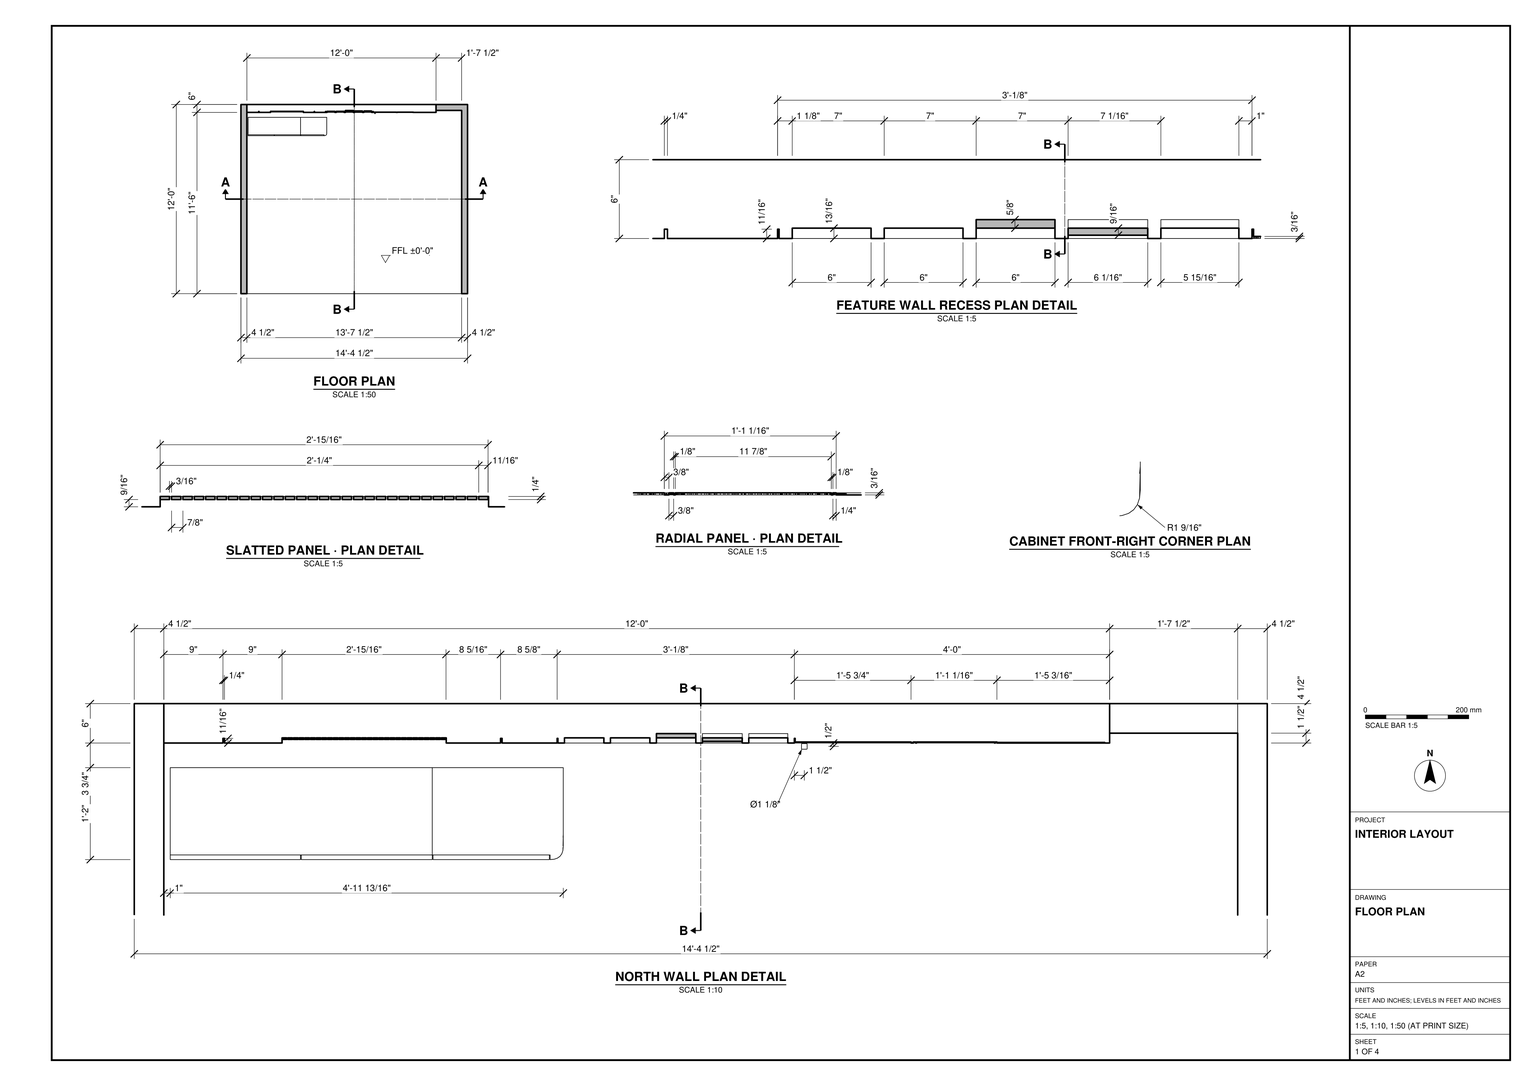
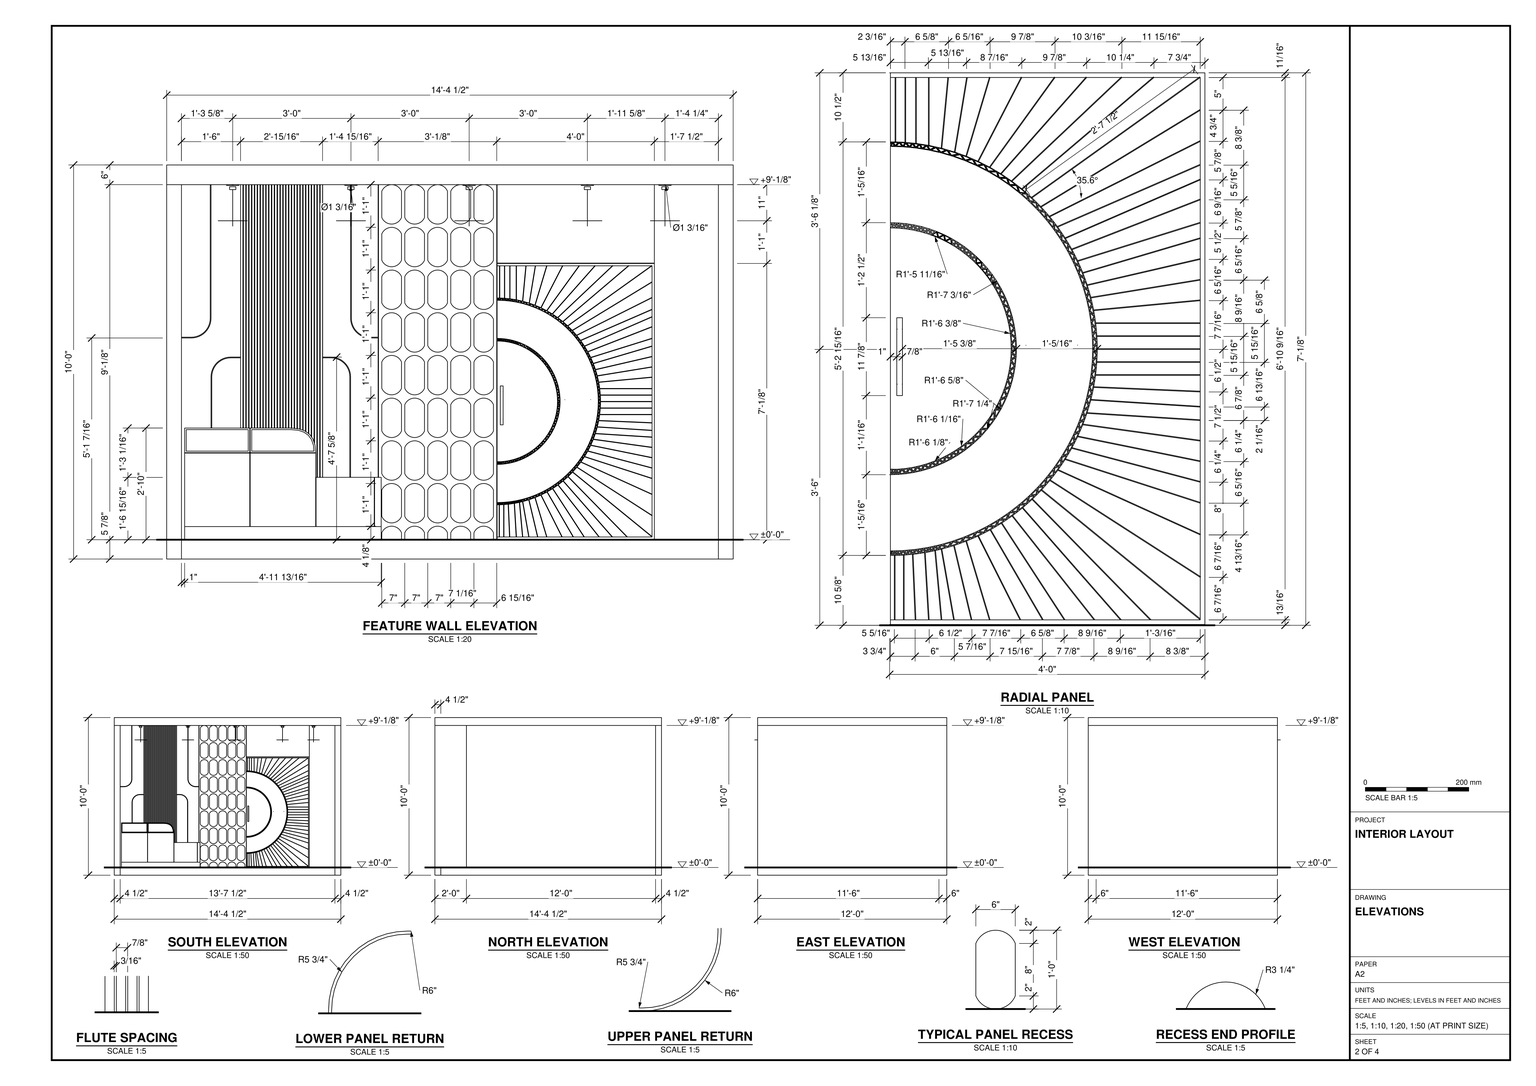
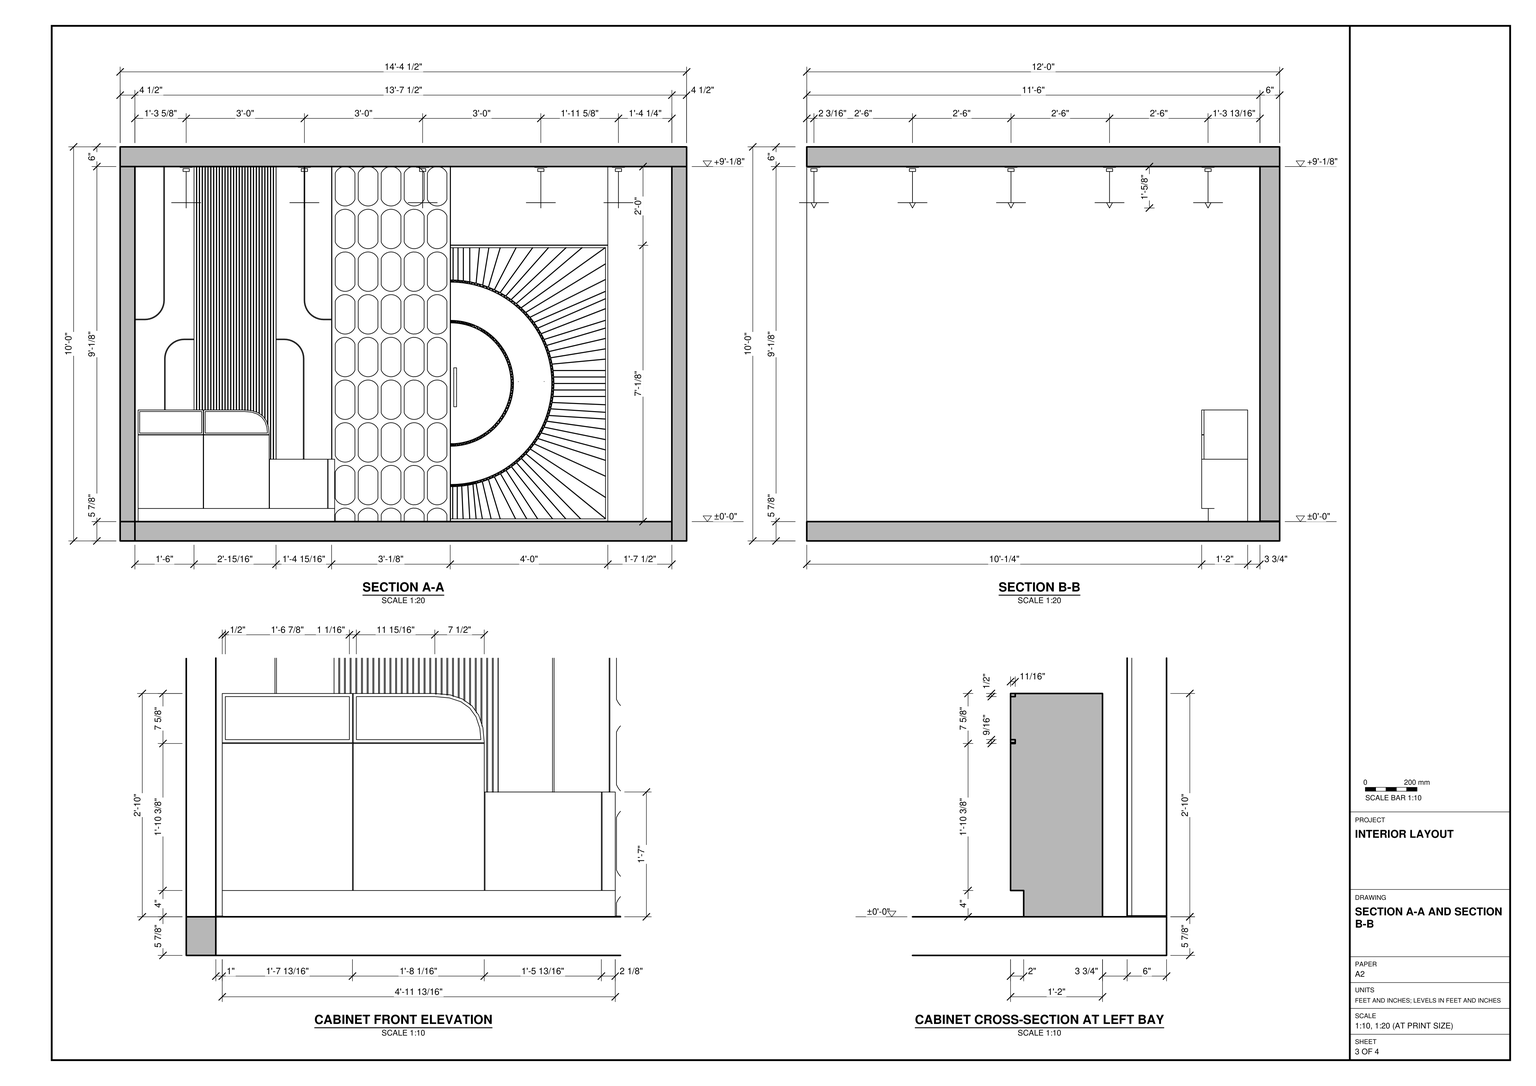
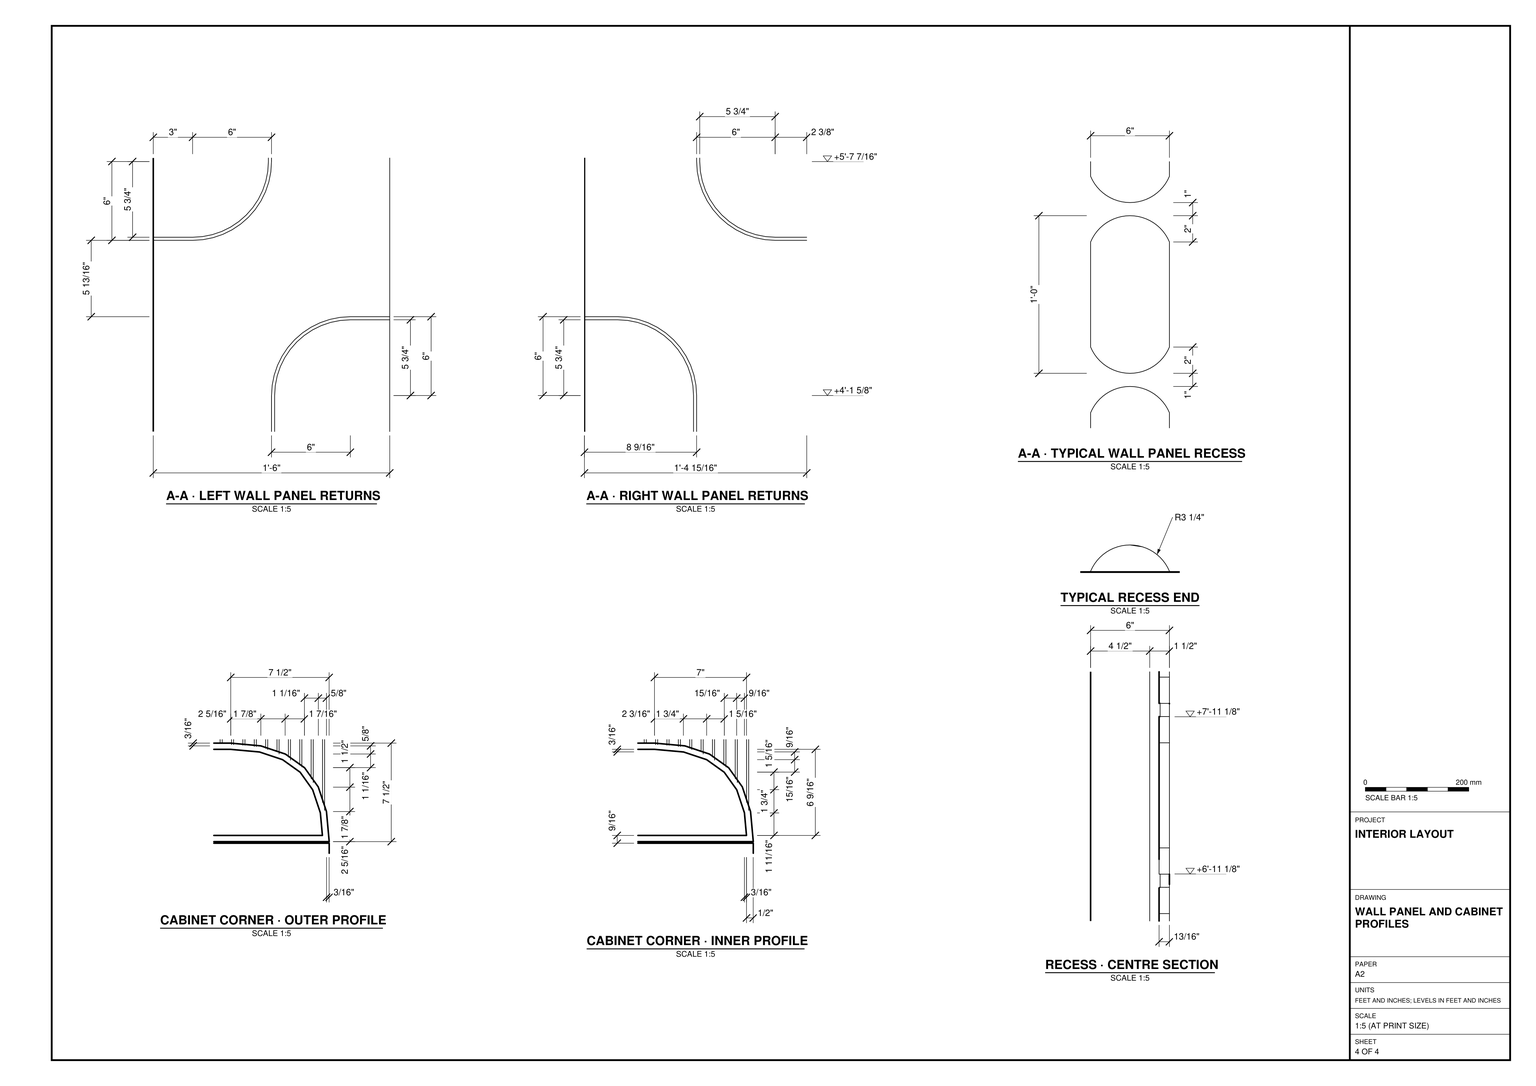
Build the interior in SketchUp from task_files/diagram_01.pdf. Work in feet and inches. The room shell is 14'-4 1/2" wide, 12'-0" deep and 10'-0" high overall, with the finished floor at ±0'-0". Model the floor slab, ceiling slab, north wall and two side walls at the thicknesses shown in plan and section. Leave the south side open so the feature wall can be seen in elevation.

Lay out the north wall from left to right. Model the narrow vertical slats and the curved returns of the adjacent panels, followed by the grid of rounded-ended recesses. Use the plan details to give these features depth. To the right of the recesses, fit the rectangular radial panel with its semicircular centre, surrounding band and divisions fanning out to the frame. Retain the plain wall above the radial panel and at its right end.

Place the stepped cabinet in front of the left-hand panels. Follow the cabinet details for its bay divisions, curved corner, recessed plinth and clearance from the wall. Position the lights as indicated in the sections. Lights, decor and loose items shown may use any suitable library components. Keep the shell elements and individual joinery pieces in separate groups or components, using components for repeated parts. Save one SketchUp model as output_files/room_with_a_feature_wall_and_stepped_cabinet.skp.

# SketchUp Ruby script. Lengths in inches.
U = 1.inch
M = Sketchup.active_model
def pt(a) = Geom::Point3d.new(a.map { |v| v * U })
def face(e, loops, mat)
  f = e.add_face(loops[0].map { |a| pt(a) })
  loops[1..].each { |l| e.add_face(l.map { |a| pt(a) }).erase! }
  f.material = f.back_material = mat if mat
  f
end
# faces: each face lists its corners as indices into pts; further lists are holes
def faces(e, pts, list, mat = nil) = list.each { |f| face(e, (f[0].is_a?(Array) ? f : [f]).map { |l| l.map { |i| pts[i] } }, mat) }
# xy, xz, yz: faces in a plane at the given z, y or x. An outline is a flat list of corners, or four numbers for a rectangle; further outlines are holes
def ring(l) = l.size == 4 ? [[l[0], l[1]], [l[2], l[1]], [l[2], l[3]], [l[0], l[3]]] : l.each_slice(2).to_a
def flat(e, list, mat, &to3) = list.each { |f| face(e, (f[0].is_a?(Array) ? f : [f]).map { |l| ring(l).map { |u, v| to3.(u, v) } }, mat) }
def xy(e, z, list, mat = nil) = flat(e, list, mat) { |x, y| [x, y, z] }
def xz(e, y, list, mat = nil) = flat(e, list, mat) { |x, z| [x, y, z] }
def yz(e, x, list, mat = nil) = flat(e, list, mat) { |y, z| [x, y, z] }
def lines(e, pts, list) = list.each { |a, b| e.add_line(pt(pts[a]), pt(pts[b])) }
# prism: a flat outline (further loops are holes) pulled along v
def prism(e, loops, v, mat = nil)
  f = face(e, loops, mat); d = Geom::Vector3d.new(v.map { |x| x * U })
  f.pushpull(f.normal.samedirection?(d) ? d.length : -d.length)
end
def box(e, o, s, mat = nil) = prism(e, [[o, [o[0] + s[0], o[1], o[2]], [o[0] + s[0], o[1] + s[1], o[2]], [o[0], o[1] + s[1], o[2]]]], [0, 0, s[2]], mat)
def at(x, y, z, deg = 0) = Geom::Transformation.translation(pt([x, y, z])) * Geom::Transformation.rotation(ORIGIN, Z_AXIS, deg.degrees)
def axes(o, x, y, z) = Geom::Transformation.new([*x, 0, *y, 0, *z, 0, *pt(o).to_a, 1])
def part(name) = M.definitions.add(name)
# library, detail: a bought-in or finely detailed component or shape, given as its bounding box
def library(name, o, s) = part(name).tap { |d| box(d.entities, o, s) }
def detail(e, o, s) = box(e.add_group.entities, o, s)
def put(e, d, t, mat = nil) = e.add_instance(d, t).tap { |i| i.material = mat if mat }
def group(e, t, mat = nil) = e.add_group.tap { |g| g.transformation = t; g.material = mat if mat }.entities
root = M.entities
M.materials.add("Tafisa-Gardenia-or-Gardenia-PM775-4K").color = [246, 245, 235]
M.materials.add("Uniboard-L19-Putty-4K").color = [187, 181, 160]
M.materials.add("[Color M09]").color = [0, 0, 0]
c1 = part("Group194\#1")
p = [[0,0,0],[0,0,-16.77],[-0.04,0,-16.77],[0.28,-54,0],[-0.28,-54,0],[0.28,54,0],
  [0.28,0,0],[-0.28,54,0],[0.04,0,-16.77],[-0.28,0,0],[0,0,-27.14]]
lines(c1.entities,p,[[0,1],[1,2],[3,4],[5,6],[7,5],[1,8],[9,0],[0,6],[8,10],[4,9],[6,3],[2,10],
  [9,7]])
c2 = part("Rectangle Light")
put(c2.entities,c1,at(0,0,0))
c3 = part("Group196\#1")
p = [[0,0,0],[0,0,-16.77],[-0.04,0,-16.77],[0.28,-54,0],[-0.28,-54,0],[0.28,54,0],
  [0.28,0,0],[-0.28,54,0],[0.04,0,-16.77],[-0.28,0,0],[0,0,-27.14]]
lines(c3.entities,p,[[0,1],[1,2],[3,4],[5,6],[7,5],[1,8],[9,0],[0,6],[8,10],[4,9],[6,3],[2,10],
  [9,7]])
c4 = part("Rectangle Light\#1")
put(c4.entities,c3,at(0,0,0))
c5 = library("Group",[0,0,0],[144,6,108])
c6 = library("Group\#8",[0,0,0],[8.9,8.9,12.62])
put(root,c2,axes([22.51,138.28,60],[0,-1,0],[0,0,-1],[-1,0,0]))
put(root,c4,axes([47.49,138.28,60],[0,-1,0],[0,0,-1],[1,0,0]))
g1 = group(root,at(4.5,0,0),"Tafisa-Gardenia-or-Gardenia-PM775-4K")
xy(g1,0,[[-4.5,0,0,144],[0,0,163.5,144],[163.5,0,168,144]])
xy(g1,5.88,[[-4.5,0,0,144],[0,0,163.5,0,163.5,139.5,144,139.5,144,144,0,144],[144,139.5,163.5,144]])
xy(g1,114,[[163.5,0,168,0,168,144,144,144,144,139.5,163.5,139.5]])
xz(g1,0,[[-4.5,0,0,5.88],[0,0,163.5,5.88],[163.5,0,168,114]])
xz(g1,139.5,[[144,5.88,163.5,114]])
xz(g1,144,[[-4.5,0,0,5.88],[0,0,163.5,5.88],[163.5,0,163.5,5.88,144,5.88,144,114,168,114,168,0]])
yz(g1,-4.5,[[0,0,144,5.88]])
yz(g1,0,[[0,0,144,5.88]])
yz(g1,144,[[139.5,5.88,144,114]])
yz(g1,163.5,[[0,0,144,5.88],[0,5.88,139.5,114]])
yz(g1,168,[[0,0,144,114]])
put(root,c5,at(4.5,138,6))
g2 = group(root,at(101.59,137.06,52.7))
xy(g2,-11.84,[[0.09,0,0.04,0.01,0.01,0.04,0,0.09,0,0.77,0.01,0.8125,0.04,0.85,0.09,0.86,0.77,0.86,0.8125,0.85,0.85,0.8125,0.86,0.77,0.86,0.09,0.85,0.04,0.81,0.01,0.77,0]],"[Color M09]")
xy(g2,-10.1,[[0,0.45,0.86,0.45,0.86,0.77,0.85,0.8125,0.8125,0.85,0.77,0.86,0.09,0.86,0.04,0.85,0.01,0.8125,0,0.77]],"[Color M09]")
xy(g2,-1.72,[[0,0.45,0,0.77,0.01,0.8125,0.04,0.85,0.09,0.86,0.77,0.86,0.8125,0.85,0.85,0.8125,0.86,0.77,0.86,0.45]],"[Color M09]")
xy(g2,0.02,[[0.09,0,0.77,0,0.81,0.01,0.85,0.04,0.86,0.09,0.86,0.77,0.85,0.8125,0.8125,0.85,0.77,0.86,0.09,0.86,0.04,0.85,0.01,0.8125,0,0.77,0,0.09,0.01,0.04,0.04,0.01]],"[Color M09]")
xz(g2,0,[[0.09,-11.84,0.77,0.02]],"[Color M09]")
xz(g2,0.26,[[0,-9.91,0.86,-1.91]],"[Color M09]")
xz(g2,0.86,[[0.09,-11.84,0.77,-10.1],[0.09,-1.72,0.77,0.02]],"[Color M09]")
yz(g2,0,[[0.09,-11.84,0.09,0.02,0.77,0.02,0.77,-1.72,0.45,-1.72,0.36,-1.75,0.29,-1.82,0.26,-1.91,0.26,-9.91,0.29,-10.01,0.36,-10.07,0.45,-10.1,0.77,-10.1,0.77,-11.84]],"[Color M09]")
yz(g2,0.86,[[0.09,-11.84,0.77,-11.84,0.77,-10.1,0.45,-10.1,0.36,-10.07,0.29,-10.01,0.26,-9.91,0.26,-1.91,0.29,-1.82,0.36,-1.75,0.45,-1.72,0.77,-1.72,0.77,0.02,0.09,0.02]],"[Color M09]")
p = [[0.04,0.01,-11.84],[0.09,0,-11.84],[0.09,0,0.02],[0.04,0.01,0.02],[0.01,0.04,-11.84],[0.01,0.04,0.02],
  [0,0.09,0.02],[0,0.09,-11.84],[0.85,0.04,-11.84],[0.85,0.04,0.02],[0.81,0.01,0.02],[0.81,0.01,-11.84],
  [0.77,0,-11.84],[0.77,0,0.02],[0.86,0.09,-11.84],[0.86,0.09,0.02],[0.01,0.8125,-11.84],[0,0.77,-11.84],
  [0,0.77,-10.1],[0.01,0.8125,-10.1],[0.04,0.85,-11.84],[0.04,0.85,-10.1],[0.09,0.86,-11.84],[0.09,0.86,-10.1],
  [0.8125,0.85,-11.84],[0.77,0.86,-11.84],[0.77,0.86,-10.1],[0.8125,0.85,-10.1],[0.85,0.8125,-11.84],[0.85,0.8125,-10.1],
  [0.86,0.77,-11.84],[0.86,0.77,-10.1],[0.86,0.29,-10.01],[0.86,0.36,-10.07],[0,0.36,-10.07],[0,0.29,-10.01],
  [0.86,0.45,-10.1],[0,0.45,-10.1],[0.86,0.26,-9.91],[0,0.26,-9.91],[0,0.29,-1.82],[0.86,0.29,-1.82],
  [0.86,0.26,-1.91],[0,0.26,-1.91],[0.86,0.36,-1.75],[0,0.36,-1.75],[0.86,0.45,-1.72],[0,0.45,-1.72],
  [0,0.77,-1.72],[0,0.77,0.02],[0.01,0.8125,0.02],[0.01,0.8125,-1.72],[0.04,0.85,0.02],[0.09,0.86,0.02],
  [0.09,0.86,-1.72],[0.04,0.85,-1.72],[0.77,0.86,0.02],[0.8125,0.85,0.02],[0.8125,0.85,-1.72],[0.77,0.86,-1.72],
  [0.85,0.8125,-1.72],[0.85,0.8125,0.02],[0.86,0.77,0.02],[0.86,0.77,-1.72]]
faces(g2,p,[[0,1,2,3],[4,0,3,5],[4,5,6,7],[8,9,10,11],[12,11,10,13],[14,15,9,8],[16,17,18,19],[20,16,19,21],
  [22,20,21,23],[24,25,26,27],[28,24,27,29],[30,28,29,31],[32,33,34,35],[33,36,37,34],[38,32,35,39],[40,41,42,43],
  [44,41,40,45],[46,44,45,47],[48,49,50,51],[52,53,54,55],[51,50,52,55],[56,57,58,59],[60,61,62,63],[57,61,60,58]],"[Color M09]")
g3 = group(root,at(0,0,5.88))
box(g3,[0,0,0],[4.5,144,108.12])
g4 = group(root,at(5.48,120.25,5.88),"Tafisa-Gardenia-or-Gardenia-PM775-4K")
xy(g4,0,[[0,2,0,14,59.84,14,59.84,3.8125,59.79,3.26,59.64,2.81,59.39,2.45,59.03,2.2,58.58,2.05,58.02,2]])
xy(g4,4,[[0,0,0,2,19.95,2,19.95,0.71,19.83,0.71,19.83,0],[19.95,0,39.89,0.71],[57.84,0,57.84,0.71,39.89,0.71,39.89,2,58.02,2,58.58,2.05,59.03,2.2,59.39,2.45,59.64,2.81,59.79,3.26,59.84,3.8125,59.78,1.39,59.62,0.89,59.34,0.5,58.95,0.22,58.45,0.06],[40.01,0,57.72,0.71],[19.95,0.71,39.89,2]])
xy(g4,19,[[40.01,0,57.72,0.71]])
xy(g4,19,[[57.84,0,58.45,0.06,58.95,0.22,59.34,0.5,59.62,0.89,59.78,1.39,59.84,2,59.84,14,39.89,14,39.89,0.71,57.84,0.71]],"Uniboard-L19-Putty-4K")
xy(g4,26.38,[[0,0,19.83,0.71],[19.95,0,39.89,0.71]])
xy(g4,26.5,[[0,0,19.83,0.71],[19.95,0,39.89,0.71]])
xy(g4,26.97,[[0.47,0,19.36,0.71],[20.42,0,39.375,0.71]])
xy(g4,33.53,[[0.47,0,19.36,0.71],[20.42,0,32.37,0.71]])
xy(g4,34,[[0,0,19.83,0.71],[19.95,0,32.39,0.71]])
xy(g4,34,[[0,0.71,32.39,14]],"Uniboard-L19-Putty-4K")
xz(g4,0,[[0,4,19.83,26.38],[19.95,4,39.89,26.38],[40.01,4,57.72,19],[0.47,26.97,19.36,33.53],[20.42,26.97,39.375,26.97,39.22,28.69,38.63,30.45,37.68,31.79,36.34,32.74,34.59,33.33,32.37,33.53,20.42,33.53]])
xz(g4,0,[[[0,26.5,19.83,34],[0.47,26.97,19.36,33.53]],[[19.95,26.5,39.89,26.5,39.68,28.79,39.06,30.67,38.02,32.125,36.56,33.17,34.68,33.79,32.39,34,19.95,34],[20.42,26.97,20.42,33.53,32.37,33.53,34.59,33.33,36.34,32.74,37.68,31.79,38.63,30.45,39.22,28.69,39.375,26.97]]],"Uniboard-L19-Putty-4K")
xz(g4,0.71,[[19.83,4,19.95,26.38],[19.95,4,39.89,26.38],[39.89,4,40.01,19],[40.01,4,57.72,19],[57.72,4,57.84,19],
  [0,26.38,19.95,26.5],[19.95,26.38,39.89,26.5],[[0,26.5,19.83,34],[0.47,26.97,19.36,33.53]],[[19.95,26.5,19.95,34,32.39,34,34.68,33.79,36.56,33.17,38.02,32.125,39.06,30.67,39.68,28.79,39.89,26.5],[20.42,26.97,39.375,26.97,39.22,28.69,38.63,30.45,37.68,31.79,36.34,32.74,34.59,33.33,32.37,33.53,20.42,33.53]]])
xz(g4,0.71,[[19.83,26.5,19.95,34]],"Uniboard-L19-Putty-4K")
xz(g4,2,[[0,0,58.02,4]],"Uniboard-L19-Putty-4K")
xz(g4,14,[[0,0,0,34,32.39,34,34.68,33.79,36.56,33.17,38.02,32.125,39.06,30.67,39.68,28.79,39.89,26.5,39.89,19,59.84,19,59.84,0]])
yz(g4,0,[[2,0,2,4,0,4,0,26.38,0.71,26.38,0.71,34,14,34,14,0],[0,26.5,0.71,34]])
yz(g4,0.47,[[0,26.97,0.71,33.53]])
yz(g4,19.36,[[0,26.97,0.71,33.53]])
yz(g4,19.83,[[0,4,0.71,26.38]])
yz(g4,19.83,[[0,26.5,0.71,34]],"Uniboard-L19-Putty-4K")
yz(g4,19.95,[[0,4,0.71,26.38],[0,26.5,0.71,34]])
yz(g4,20.42,[[0,26.97,0.71,33.53]])
yz(g4,39.89,[[0,4,0.71,19],[0,19,0.71,26.38]])
yz(g4,39.89,[[0.71,19,14,26.5]],"Uniboard-L19-Putty-4K")
yz(g4,40.01,[[0,4,0.71,19]])
yz(g4,57.72,[[0,4,0.71,19]])
yz(g4,57.84,[[0,4,0.71,19]])
yz(g4,59.84,[[3.8125,0,14,0,14,19,2,19,2,4,3.8125,4]],"Uniboard-L19-Putty-4K")
p = [[58.58,2.05,0],[58.58,2.05,4],[58.02,2,4],[58.02,2,0],[59.03,2.2,0],[59.03,2.2,4],
  [59.39,2.45,0],[59.39,2.45,4],[59.64,2.81,0],[59.64,2.81,4],[59.79,3.26,0],[59.79,3.26,4],
  [59.84,3.8125,0],[59.84,3.8125,4],[57.84,0,19],[57.84,0,4],[58.45,0.06,4],[58.45,0.06,19],
  [58.95,0.22,4],[58.95,0.22,19],[59.34,0.5,4],[59.34,0.5,19],[59.62,0.89,4],[59.62,0.89,19],
  [59.78,1.39,4],[59.78,1.39,19],[59.84,2,4],[59.84,2,19],[39.68,0.71,28.79],[39.68,0,28.79],
  [39.89,0,26.5],[39.89,0.71,26.5],[39.68,14,28.79],[39.89,14,26.5],[39.375,0.71,26.97],[39.375,0,26.97],
  [39.22,0,28.69],[39.22,0.71,28.69],[38.63,0,30.45],[38.63,0.71,30.45],[39.06,0.71,30.67],[39.06,0,30.67],
  [39.06,14,30.67],[37.68,0,31.79],[37.68,0.71,31.79],[38.02,0.71,32.125],[38.02,0,32.125],[38.02,14,32.125],
  [36.34,0,32.74],[36.34,0.71,32.74],[36.56,0.71,33.17],[36.56,0,33.17],[36.56,14,33.17],[34.59,0,33.33],
  [34.59,0.71,33.33],[34.68,0.71,33.79],[34.68,0,33.79],[34.68,14,33.79],[32.37,0,33.53],[32.37,0.71,33.53],
  [32.39,0.71,34],[32.39,0,34],[32.39,14,34]]
faces(g4,p,[[0,1,2,3],[4,5,1,0],[6,7,5,4],[8,9,7,6],[10,11,9,8],[12,13,11,10],[14,15,16,17],[17,16,18,19],
  [19,18,20,21],[21,20,22,23],[23,22,24,25],[25,24,26,27],[32,28,31,33],[42,40,28,32],[47,45,40,42],[52,50,45,47],
  [57,55,50,52],[62,60,55,57]],"Uniboard-L19-Putty-4K")
faces(g4,p,[[28,29,30,31],[34,35,36,37],[37,36,38,39],[40,41,29,28],[39,38,43,44],[45,46,41,40],[44,43,48,49],[50,51,46,45],
  [49,48,53,54],[55,56,51,50],[54,53,58,59],[60,61,56,55]])
g5 = group(root,at(0,0,114))
box(g5,[0,0,0],[172.5,144,6])
put(root,c6,at(15.66,117.74,101.38))
put(root,c6,at(51.66,117.74,101.38))
put(root,c6,at(87.66,117.74,101.38))
put(root,c6,at(123.66,117.74,101.38))
put(root,c6,at(147.28,117.74,101.38))
put(root,c6,at(51.66,87.74,101.38))
put(root,c6,at(123.66,87.74,101.38))
put(root,c6,at(15.66,87.74,101.38))
put(root,c6,at(87.66,87.74,101.38))
put(root,c6,at(147.28,87.74,101.38))
put(root,c6,at(51.66,57.74,101.38))
put(root,c6,at(123.66,57.74,101.38))
put(root,c6,at(15.66,57.74,101.38))
put(root,c6,at(87.66,57.74,101.38))
put(root,c6,at(147.28,57.74,101.38))
put(root,c6,at(51.66,27.74,101.38))
put(root,c6,at(123.66,27.74,101.38))
put(root,c6,at(15.66,27.74,101.38))
put(root,c6,at(87.66,27.74,101.38))
put(root,c6,at(147.28,27.74,101.38))
put(root,c6,at(51.66,-2.26,101.38))
put(root,c6,at(123.66,-2.26,101.38))
put(root,c6,at(15.66,-2.26,101.38))
put(root,c6,at(87.66,-2.26,101.38))
put(root,c6,at(147.28,-2.26,101.38))
